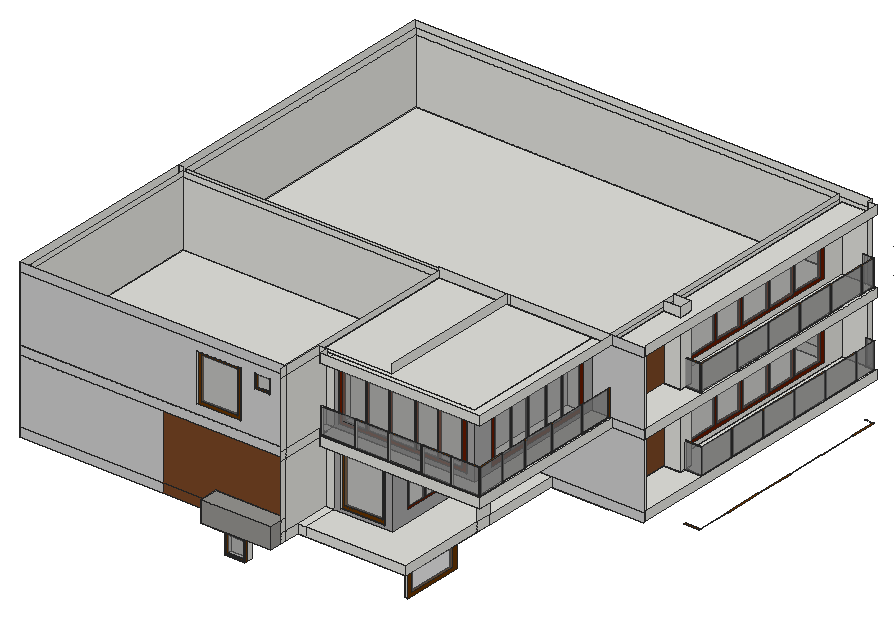
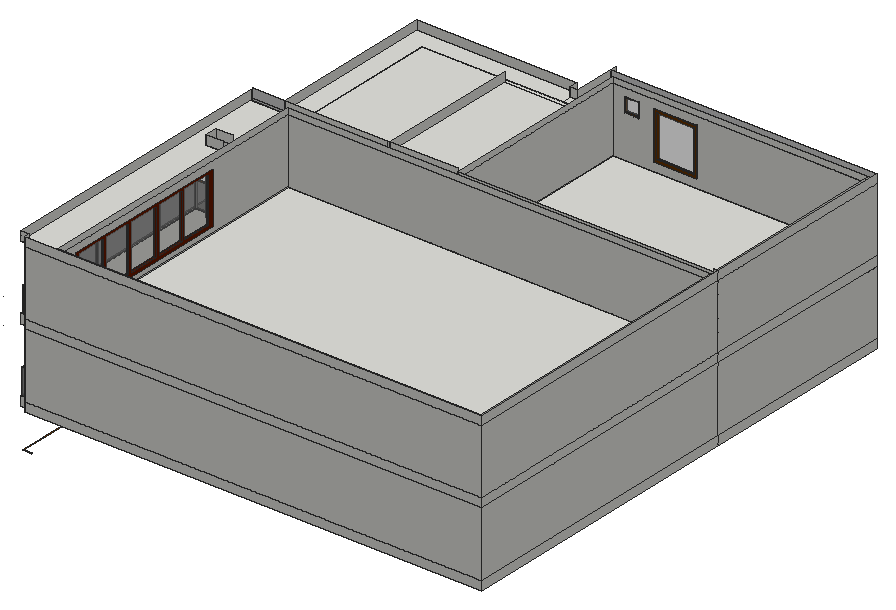
# SketchUp Ruby script. Lengths in inches.
U = 1.inch
M = Sketchup.active_model
def pt(a) = Geom::Point3d.new(a.map { |v| v * U })
def face(e, loops, mat)
  f = e.add_face(loops[0].map { |a| pt(a) })
  loops[1..].each { |l| e.add_face(l.map { |a| pt(a) }).erase! }
  f.material = f.back_material = mat if mat
  f
end
# faces: each face lists its corners as indices into pts; further lists are holes
def faces(e, pts, list, mat = nil) = list.each { |f| face(e, (f[0].is_a?(Array) ? f : [f]).map { |l| l.map { |i| pts[i] } }, mat) }
# xy, xz, yz: faces in a plane at the given z, y or x. An outline is a flat list of corners, or four numbers for a rectangle; further outlines are holes
def ring(l) = l.size == 4 ? [[l[0], l[1]], [l[2], l[1]], [l[2], l[3]], [l[0], l[3]]] : l.each_slice(2).to_a
def flat(e, list, mat, &to3) = list.each { |f| face(e, (f[0].is_a?(Array) ? f : [f]).map { |l| ring(l).map { |u, v| to3.(u, v) } }, mat) }
def xy(e, z, list, mat = nil) = flat(e, list, mat) { |x, y| [x, y, z] }
def xz(e, y, list, mat = nil) = flat(e, list, mat) { |x, z| [x, y, z] }
def yz(e, x, list, mat = nil) = flat(e, list, mat) { |y, z| [x, y, z] }
def lines(e, pts, list) = list.each { |a, b| e.add_line(pt(pts[a]), pt(pts[b])) }
# prism: a flat outline (further loops are holes) pulled along v
def prism(e, loops, v, mat = nil)
  f = face(e, loops, mat); d = Geom::Vector3d.new(v.map { |x| x * U })
  f.pushpull(f.normal.samedirection?(d) ? d.length : -d.length)
end
def box(e, o, s, mat = nil) = prism(e, [[o, [o[0] + s[0], o[1], o[2]], [o[0] + s[0], o[1] + s[1], o[2]], [o[0], o[1] + s[1], o[2]]]], [0, 0, s[2]], mat)
def at(x, y, z, deg = 0) = Geom::Transformation.translation(pt([x, y, z])) * Geom::Transformation.rotation(ORIGIN, Z_AXIS, deg.degrees)
def axes(o, x, y, z) = Geom::Transformation.new([*x, 0, *y, 0, *z, 0, *pt(o).to_a, 1])
def part(name) = M.definitions.add(name)
# library, detail: a bought-in or finely detailed component or shape, given as its bounding box
def library(name, o, s) = part(name).tap { |d| box(d.entities, o, s) }
def detail(e, o, s) = box(e.add_group.entities, o, s)
def put(e, d, t, mat = nil) = e.add_instance(d, t).tap { |i| i.material = mat if mat }
def group(e, t, mat = nil) = e.add_group.tap { |g| g.transformation = t; g.material = mat if mat }.entities
root = M.entities
M.materials.add("[Carrera Marble]").color = [207, 207, 207]
M.materials.add("[Color B08]").color = [102, 25, 0]
M.materials.add("[Color C08]").color = [102, 51, 0]
M.materials.add("[Granite Light Gray]").color = [149, 148, 144]
M.materials.add("[Stone Vein Gray]").color = [166, 165, 165]
M.materials.add("[Translucent Glass Gray]").color = [128, 128, 128]
M.materials["[Translucent Glass Gray]"].alpha = 0.5
M.materials.add("[Wood Veneer 01]").color = [120, 70, 37]
c1 = part("Group\#1")
xy(c1.entities,0,[[0,0,21.625,260.4375]],"[Color C08]")
xy(c1.entities,20.42,[[0,20.42,21.625,240.02]],"[Color C08]")
xy(c1.entities,312.95,[[0,20.42,21.625,240.02]],"[Color C08]")
xy(c1.entities,333.375,[[0,0,21.625,260.4375]],"[Color C08]")
xz(c1.entities,0,[[0,0,21.625,333.375]],"[Color C08]")
xz(c1.entities,20.42,[[0,20.42,21.625,312.95]],"[Color C08]")
xz(c1.entities,240.02,[[0,20.42,21.625,312.95]],"[Color C08]")
xz(c1.entities,260.4375,[[0,0,21.625,333.375]],"[Color C08]")
yz(c1.entities,0,[[[0,0,260.4375,333.375],[20.42,20.42,240.02,312.95]]],"[Color C08]")
yz(c1.entities,21.625,[[[0,0,260.4375,333.375],[20.42,20.42,240.02,312.95]]],"[Color C08]")
yz(c1.entities,21.625,[[20.42,20.42,240.02,312.95]],"[Translucent Glass Gray]")
c2 = part("Group\#3")
xy(c2.entities,0,[[0,0,23.0625,440.625]],"[Color B08]")
xy(c2.entities,14.28,[[0,14.28,23.0625,92.65],[0,98.4,23.0625,173.71],[0,179.46,23.0625,261.65],[0,267.4,23.0625,340.59],[0,346.34,23.0625,426.35]],"[Color B08]")
xy(c2.entities,204.03,[[0,14.28,23.0625,92.65],[0,98.4,23.0625,173.71],[0,179.46,23.0625,261.65],[0,267.4,23.0625,340.59],[0,346.34,23.0625,426.35]],"[Color B08]")
xy(c2.entities,218.3125,[[0,0,23.0625,440.625]],"[Color B08]")
xz(c2.entities,0,[[0,0,23.0625,218.3125]],"[Color B08]")
xz(c2.entities,14.28,[[0,14.28,23.0625,204.03]],"[Color B08]")
xz(c2.entities,92.65,[[0,14.28,23.0625,204.03]],"[Color B08]")
xz(c2.entities,98.4,[[0,14.28,23.0625,204.03]],"[Color B08]")
xz(c2.entities,173.71,[[0,14.28,23.0625,204.03]],"[Color B08]")
xz(c2.entities,179.46,[[0,14.28,23.0625,204.03]],"[Color B08]")
xz(c2.entities,261.65,[[0,14.28,23.0625,204.03]],"[Color B08]")
xz(c2.entities,267.4,[[0,14.28,23.0625,204.03]],"[Color B08]")
xz(c2.entities,340.59,[[0,14.28,23.0625,204.03]],"[Color B08]")
xz(c2.entities,346.34,[[0,14.28,23.0625,204.03]],"[Color B08]")
xz(c2.entities,426.35,[[0,14.28,23.0625,204.03]],"[Color B08]")
xz(c2.entities,440.625,[[0,0,23.0625,218.3125]],"[Color B08]")
yz(c2.entities,0,[[[0,0,440.625,218.3125],[179.46,14.28,261.65,204.03],[346.34,14.28,426.35,204.03],[14.28,14.28,92.65,204.03],[98.4,14.28,173.71,204.03],[267.4,14.28,340.59,204.03]]],"[Color B08]")
yz(c2.entities,23.0625,[[[0,0,440.625,218.3125],[179.46,14.28,261.65,204.03],[346.34,14.28,426.35,204.03],[14.28,14.28,92.65,204.03],[98.4,14.28,173.71,204.03],[267.4,14.28,340.59,204.03]]],"[Color B08]")
yz(c2.entities,23.0625,[[14.28,14.28,92.65,204.03],[98.4,14.28,173.71,204.03],[179.46,14.28,261.65,204.03],[267.4,14.28,340.59,204.03],[346.34,14.28,426.35,204.03]],"[Translucent Glass Gray]")
xy(root,566.178,[[607.75,336.9375,613.75,449.375]])
xy(root,603,[[828.5625,706.6875,856.375,711.1875],[856.375,706.6875,857.6875,711.1875],[856.375,711.1875,857.6875,772.085],[856.375,772.085,857.6875,773.74],[856.375,773.74,857.6875,844.71],
  [856.375,844.71,857.6875,846.365],[856.375,846.365,857.6875,917.335],[856.375,917.335,857.6875,918.99],[856.375,918.99,857.6875,989.96],[856.375,989.96,857.6875,991.615],
  [856.375,991.615,857.6875,1062.585],[856.375,1062.585,857.6875,1064.24],[856.375,1064.24,857.6875,1110],[841.515,1110,856.375,1110.8125],[856.375,1110,857.6875,1110.8125]],"[Color C08]")
xy(root,638.3125,[[406.64,171.6875,444.077,187]])
xy(root,659.99,[[607.75,336.9375,613.75,449.375]])
xy(root,661.371,[[791.375,750.158,797.375,1072.783]])
xy(root,667.778,[[517.666,301.1875,599.791,308.3125]])
xy(root,669,[[9,579,791.375,1111.6875]])
xy(root,675,[[9,579,791.375,1111.6875],[797.375,579,797.375,699.063,828.5625,699.063,828.5625,723.022,797.375,723.022,797.375,1111.6875,861.375,1111.6875,861.375,579]])
xy(root,675.75,[[362.246,171.6875,362.246,207.0625,491.3125,207.0625,491.3125,171.6875,444.077,171.6875,444.077,187,406.64,187,406.64,171.6875],[406.64,171.6875,444.077,187],[0,207.0625,0,573,9,573,9,213.0625,482.6875,213.0625,482.6875,308.3125,607.75,308.3125,607.75,573,613.75,573,613.75,301.1875,491.3125,301.1875,491.3125,207.0625],[491.3125,235.5625,506.0625,301.1875],[506.0625,235.5625,506.0625,301.1875,613.75,301.1875,613.75,573,691.028,573,691.028,235.5625]])
xy(root,686,[[9,213.0625,9,573,607.75,573,607.75,308.3125,482.6875,308.3125,482.6875,213.0625]])
xy(root,692,[[0,207.0625,0,573,9,573,9,213.0625,482.6875,213.0625,482.6875,308.3125,607.75,308.3125,607.75,573,613.75,573,613.75,301.1875,491.3125,301.1875,491.3125,207.0625],[9,213.0625,482.6875,213.0625,482.6875,308.3125,607.75,308.3125,607.75,573,9,573],[491.3125,235.5625,506.0625,301.1875],[506.0625,235.5625,691.028,235.5625,691.028,573,613.75,573,613.75,301.1875,506.0625,301.1875],[797.375,579,861.375,579,861.375,1111.6875,797.375,1111.6875,797.375,723.022,828.5625,723.022,828.5625,710.721,858.375,710.721,858.375,1109.6875,843.51,1109.6875,843.51,1110.875,859.875,1110.875,859.875,708.846,828.5625,708.846,828.5625,699.063,797.375,699.063],
  [828.5625,708.846,828.5625,710.721,858.375,710.721,858.375,779.522,859.875,779.522,859.875,708.846],[858.375,779.522,859.875,781.054],[858.375,781.054,859.875,851.647],[858.375,851.647,859.875,853.179],[858.375,853.179,859.875,923.772],
  [858.375,923.772,859.875,925.304],[858.375,925.304,859.875,995.897],[858.375,995.897,859.875,997.429],[858.375,997.429,859.875,1068.022],[858.375,1068.022,859.875,1069.554],
  [858.375,1069.554,858.375,1109.6875,843.51,1109.6875,843.51,1110.875,859.875,1110.875,859.875,1069.554]])
xy(root,697.447,[[517.451,301.1875,599.764,308.3125]])
xy(root,698.559,[[791.375,750.158,797.375,1072.783]])
xy(root,712.73,[[607.75,333.789,613.75,533.476]])
xy(root,714.625,[[362.246,171.6875,491.3125,207.0625]],"[Granite Light Gray]")
xy(root,740,[[828.5625,708.846,858.375,710.721],[858.375,708.846,859.875,710.721],[858.375,710.721,859.875,779.522],[858.375,779.522,859.875,781.054],[858.375,781.054,859.875,851.647],
  [858.375,851.647,859.875,853.179],[858.375,853.179,859.875,923.772],[858.375,923.772,859.875,925.304],[858.375,925.304,859.875,995.897],[858.375,995.897,859.875,997.429],
  [858.375,997.429,859.875,1068.022],[858.375,1068.022,859.875,1069.554],[858.375,1069.554,859.875,1069.554,859.875,1110.875,843.51,1110.875,843.51,1109.6875,858.375,1109.6875]],"[Color C08]")
xy(root,789.667,[[607.75,333.789,613.75,533.476]])
xy(root,797.434,[[791.375,750.158,797.375,1072.783]])
xy(root,800.572,[[517.451,301.1875,599.764,308.3125]])
xy(root,812,[[0,207.0625,0,573,9,573,9,213.0625,482.6875,213.0625,482.6875,308.3125,607.75,308.3125,607.75,573,613.75,573,613.75,301.1875,491.3125,301.1875,491.3125,207.0625],[[506.0625,267.5625,506.0625,301.1875,613.75,301.1875,613.75,573,801.71,573,801.71,267.5625],[691.028,400.901,719.841,429.151]],[491.3125,282.8125,506.0625,301.1875],[482.6875,308.3125,607.75,573],[691.028,400.901,719.841,429.151],
  [797.375,579,797.375,699.063,828.5625,699.063,828.5625,723.022,797.375,723.022,797.375,1111.6875,861.375,1111.6875,861.375,579]])
xy(root,822.125,[[9,213.0625,482.6875,573]])
xy(root,823,[[9,579,791.375,1111.6875]])
xy(root,829,[[0,207.0625,0,573,9,573,9,213.0625,482.6875,213.0625,482.6875,308.3125,607.75,308.3125,607.75,573,766.0625,573,766.0625,301.1875,491.3125,301.1875,491.3125,207.0625],[9,213.0625,482.6875,573],[506.0625,267.5625,801.71,267.5625,801.71,573,799.585,573,799.573,569.893,799.355,508.877,799.351,507.635,799.148,440.495,799.141,438.54,798.945,378.961,798.937,376.525,798.772,326.426,798.772,324.775,799.585,272.6875,799.585,270.6875,506.0625,270.6875],[506.0625,270.6875,508.257,272.6875],[508.257,270.6875,567.823,272.6875],
  [567.823,270.6875,569.893,272.6875],[569.893,270.6875,629.323,272.6875],[629.323,270.6875,631.393,272.6875],[631.393,270.6875,691.636,272.6875],[691.636,270.6875,693.706,272.6875],
  [693.706,270.6875,746.198,272.6875],[746.198,270.6875,748.268,272.6875],[748.268,270.6875,797.585,272.6875],[797.585,270.6875,797.779,272.6875],[797.779,270.6875,799.585,272.375],
  [797.779,272.375,799.585,272.6875],[506.0625,272.6875,691.636,272.6875,691.636,272.75,693.706,272.75,693.706,272.6875,797.585,272.6875,797.585,376.529,797.562,376.529,797.57,378.966,797.585,378.966,797.585,438.545,797.579,438.545,797.585,440.232,797.585,440.5,797.584,569.9,797.585,569.984,797.585,573,766.0625,573,766.0625,301.1875,506.0625,301.1875],[691.636,272.6875,693.706,272.75],[797.585,272.6875,797.585,324.775,798.772,324.775,799.585,272.6875],[491.3125,282.8125,506.0625,301.1875],
  [482.6875,308.3125,607.75,573],[797.585,324.775,798.772,326.426],[797.585,326.426,797.585,376.529,798.937,376.525,798.772,326.426],[798.937,376.525,797.585,376.529,797.585,378.966,798.945,378.961],[797.562,376.529,797.57,378.966,797.585,378.966,797.585,376.529],
  [798.945,378.961,797.585,378.966,797.585,438.545,799.141,438.54],[799.141,438.54,797.585,438.545,797.585,440.5,799.148,440.495],[797.579,438.545,797.585,438.545,797.585,440.232],[799.148,440.495,797.585,440.5,797.584,569.9,799.573,569.893,799.355,508.877,797.605,508.883,797.601,507.641,799.351,507.635],[799.351,507.635,797.601,507.641,797.605,508.883,799.355,508.877],
  [799.573,569.893,797.584,569.9,797.585,569.984,797.595,573,799.585,573],[797.585,569.984,797.585,573,797.595,573],[797.595,573,797.595,573.007,799.585,573],[9,579,791.375,1111.6875],[797.375,579,861.375,579,861.375,1111.6875,797.375,1111.6875,797.375,723.022,828.5625,723.022,828.5625,712.375,856.375,712.375,856.375,1109.385,838.579,1109.385,838.579,1110.448,858.125,1110.448,858.125,709.875,828.5625,709.875,828.5625,699.063,797.375,699.063],
  [828.5625,709.875,856.375,712.375],[856.375,709.875,858.125,712.375],[856.375,712.375,858.125,794.565],[856.375,794.565,858.125,796],[856.375,796,858.125,866.565],
  [856.375,866.565,858.125,868],[856.375,868,858.125,938.565],[856.375,938.565,858.125,940],[856.375,940,858.125,1010.565],[856.375,1010.565,858.125,1012],
  [856.375,1012,858.125,1082.565],[856.375,1082.565,858.125,1084],[856.375,1084,858.125,1109.385],[838.579,1109.385,856.375,1110.448],[856.375,1109.385,858.125,1110.448]])
xy(root,836.402,[[514.904,301.1875,750.717,325.5625]])
xy(root,836.699,[[736.6875,339.975,766.0625,551.413]])
xy(root,837.871,[[791.375,750.158,797.375,1072.783]])
xy(root,844.835,[[327.221,207.0625,407.721,213.0625]])
xy(root,877,[[691.636,272.6875,693.706,272.75],[797.562,376.529,797.585,376.529,797.585,378.966,797.57,378.966],[797.579,438.545,797.585,438.545,797.585,440.232],[797.585,569.984,797.595,573,797.585,573],[797.595,573,799.585,573,797.595,573.007]])
xy(root,877,[[506.0625,270.6875,508.257,272.6875],[508.257,270.6875,567.823,272.6875],[567.823,270.6875,569.893,272.6875],[569.893,270.6875,629.323,272.6875],[629.323,270.6875,631.393,272.6875],
  [631.393,270.6875,691.636,272.6875],[691.636,270.6875,693.706,272.6875],[693.706,270.6875,746.198,272.6875],[746.198,270.6875,748.268,272.6875],[748.268,270.6875,797.585,272.6875],
  [797.585,270.6875,799.585,272.6875],[797.585,272.6875,799.585,272.6875,798.772,324.775,797.585,324.775],[797.585,324.775,798.772,326.426],[797.585,326.426,798.772,326.426,798.937,376.525,797.585,376.529],[798.937,376.525,798.945,378.961,797.585,378.966,797.585,376.529],
  [798.945,378.961,799.141,438.54,797.585,438.545,797.585,378.966],[799.141,438.54,799.148,440.495,797.585,440.5,797.585,438.545],[799.148,440.495,799.351,507.635,797.601,507.641,797.605,508.883,799.355,508.877,799.573,569.893,797.584,569.9,797.585,440.5],[799.351,507.635,799.355,508.877,797.605,508.883,797.601,507.641],[799.573,569.893,799.585,573,797.595,573,797.585,569.984,797.584,569.9],
  [828.5625,709.875,856.375,712.375],[856.375,709.875,858.125,712.375],[856.375,712.375,858.125,794.565],[856.375,794.565,858.125,796],[856.375,796,858.125,866.565],
  [856.375,866.565,858.125,868],[856.375,868,858.125,938.565],[856.375,938.565,858.125,940],[856.375,940,858.125,1010.565],[856.375,1010.565,858.125,1012],
  [856.375,1012,858.125,1082.565],[856.375,1082.565,858.125,1084],[856.375,1084,858.125,1109.385],[838.579,1109.385,856.375,1110.448],[856.375,1109.385,858.125,1110.448]],"[Color C08]")
xy(root,907.498,[[434.387,207.0625,461.574,213.0625]])
xy(root,933.199,[[736.6875,339.975,766.0625,551.413]])
xy(root,933.96,[[327.221,207.0625,407.721,213.0625]])
xy(root,934.686,[[434.387,207.0625,461.574,213.0625]])
xy(root,936.746,[[791.375,750.158,797.375,1072.783]])
xy(root,943.152,[[514.904,301.1875,750.717,325.5625]])
xy(root,949,[[0,207.0625,0,573,9,573,9,213.0625,482.6875,213.0625,482.6875,308.3125,607.75,308.3125,607.75,573,766.0625,573,766.0625,301.1875,491.3125,301.1875,491.3125,207.0625],[506.0625,267.5625,506.0625,301.1875,766.0625,301.1875,766.0625,573,801.71,573,801.71,267.5625],[491.3125,282.8125,506.0625,301.1875],[482.6875,308.3125,607.75,573],[797.375,579,797.375,699.063,828.5625,699.063,828.5625,723.022,797.375,723.022,797.375,1111.6875,861.375,1111.6875,861.375,579]])
xz(root,171.6875,[[362.246,675.75,491.3125,714.625]],"[Granite Light Gray]")
xz(root,187,[[406.64,638.3125,444.077,675.75]])
xz(root,207.0625,[[362.246,675.75,491.3125,692],[362.246,692,491.3125,714.625]])
xz(root,207.0625,[[0,675.75,263.742,692],[0,692,263.742,812],[0,812,491.3125,829],[[0,829,491.3125,949],[327.221,844.835,407.721,933.96],[434.387,907.498,461.574,934.686]],[0,949,491.3125,966]],"[Carrera Marble]")
xz(root,207.0625,[[263.742,675.75,362.246,692],[263.742,692,362.246,692,362.246,714.625,491.3125,714.625,491.3125,812,263.742,812]],"[Wood Veneer 01]")
xz(root,213.0625,[[9,675.75,482.6875,686],[9,686,482.6875,692],[9,692,482.6875,812],[9,812,482.6875,822.125],[9,822.125,482.6875,829],
  [[9,829,482.6875,949],[327.221,844.835,407.721,933.96],[434.387,907.498,461.574,934.686]],[9,949,482.6875,960]])
xz(root,235.5625,[[491.3125,675.75,506.0625,692],[506.0625,675.75,691.028,692]])
xz(root,267.5625,[[506.0625,812,801.71,829],[506.0625,949,801.71,966]])
xz(root,270.6875,[[506.0625,829,508.257,877],[567.823,829,569.893,877],[629.323,829,631.393,877],[691.636,829,693.706,877],[746.198,829,748.268,877],
  [797.585,829,799.585,877]],"[Color C08]")
xz(root,270.6875,[[508.257,829,567.823,877],[569.893,829,629.323,877],[631.393,829,691.636,877],[693.706,829,746.198,877],[748.268,829,797.585,877]],"[Translucent Glass Gray]")
xz(root,272.6875,[[797.585,829,799.585,877]])
xz(root,272.6875,[[567.823,829,569.893,877],[629.323,829,631.393,877],[746.198,829,748.268,877]],"[Color C08]")
xz(root,272.6875,[[508.257,829,567.823,877],[569.893,829,629.323,877],[631.393,829,746.198,877],[748.268,829,797.585,877]],"[Translucent Glass Gray]")
xz(root,272.75,[[691.636,829,693.706,877]],"[Color C08]")
xz(root,282.8125,[[491.3125,812,506.0625,829],[491.3125,949,506.0625,966]])
xz(root,301.1875,[[491.3125,692,506.0625,812],[491.3125,829,506.0625,949]])
xz(root,301.1875,[[[506.0625,692,613.75,812],[517.451,697.447,599.764,800.572]],[[506.0625,829,766.0625,949],[514.904,836.402,750.717,943.152]]],"[Stone Vein Gray]")
xz(root,308.3125,[[482.6875,675.75,607.75,686],[482.6875,686,607.75,692],[[482.6875,692,607.75,812],[517.451,697.447,599.764,800.572]],[482.6875,812,607.75,829]])
xz(root,324.775,[[797.585,829,798.772,877]])
xz(root,325.5625,[[514.904,836.402,750.717,943.152]])
xz(root,326.426,[[797.585,829,798.772,877]])
xz(root,333.789,[[607.75,712.73,613.75,789.667]])
xz(root,336.9375,[[607.75,566.178,613.75,659.99]])
xz(root,339.975,[[736.6875,836.699,766.0625,933.199]])
xz(root,449.375,[[607.75,566.178,613.75,659.99]])
xz(root,533.476,[[607.75,712.73,613.75,789.667]])
xz(root,551.413,[[736.6875,836.699,766.0625,933.199]])
xz(root,573,[[0,675,9,675.75],[9,675,607.75,686],[607.75,675,613.75,675.75],[0,675.75,9,692],[607.75,675.75,691.028,692],
  [9,686,607.75,692],[0,692,9,812],[9,692,607.75,812],[607.75,692,613.75,812],[0,812,9,829],
  [9,812,482.6875,822.125],[482.6875,812,607.75,829],[607.75,812,613.75,829],[613.75,812,801.71,829],[9,822.125,482.6875,829],
  [0,829,9,949],[9,829,482.6875,949],[482.6875,829,607.75,949],[607.75,829,766.0625,949],[797.585,829,799.585,877],
  [0,949,9,966],[9,949,482.6875,960],[482.6875,949,607.75,966],[607.75,949,613.75,966],[613.75,949,801.71,966]])
xz(root,573,[[613.75,675,861.375,675,861.375,692,691.028,692,691.028,675.75,613.75,675.75],[613.75,692,861.375,812],[801.71,812,861.375,829],[766.0625,829,797.585,829,797.585,877,799.585,877,799.585,829,861.375,829,861.375,949,766.0625,949],[801.71,949,861.375,966]],"[Carrera Marble]")
xz(root,579,[[9,669,791.375,675],[9,675,791.375,692],[797.375,675,861.375,692],[9,692,791.375,812],[797.375,692,861.375,812],
  [9,812,791.375,823],[9,823,791.375,829],[9,829,791.375,949],[797.375,829,861.375,949],[9,949,791.375,960]])
xz(root,699.063,[[797.375,675,828.5625,692],[797.375,692,828.5625,812],[797.375,812,828.5625,829],[797.375,829,828.5625,949],[797.375,949,828.5625,966]])
xz(root,708.846,[[828.5625,692,859.875,740]],"[Translucent Glass Gray]")
xz(root,709.875,[[856.375,829,858.125,877]],"[Color C08]")
xz(root,709.875,[[828.5625,829,856.375,877]],"[Translucent Glass Gray]")
xz(root,710.721,[[828.5625,692,858.375,740]],"[Translucent Glass Gray]")
xz(root,712.375,[[856.375,829,858.125,877]])
xz(root,712.375,[[828.5625,829,856.375,877]],"[Translucent Glass Gray]")
xz(root,723.022,[[797.375,675,828.5625,692],[797.375,692,828.5625,812],[797.375,812,828.5625,829],[797.375,829,828.5625,949],[797.375,949,828.5625,966]])
xz(root,750.158,[[791.375,698.559,797.375,797.434],[791.375,837.871,797.375,936.746]])
xz(root,779.522,[[858.375,692,859.875,740]])
xz(root,781.054,[[858.375,692,859.875,740]])
xz(root,794.565,[[856.375,829,858.125,877]])
xz(root,796,[[856.375,829,858.125,877]])
xz(root,851.647,[[858.375,692,859.875,740]])
xz(root,853.179,[[858.375,692,859.875,740]])
xz(root,866.565,[[856.375,829,858.125,877]])
xz(root,868,[[856.375,829,858.125,877]])
xz(root,923.772,[[858.375,692,859.875,740]])
xz(root,925.304,[[858.375,692,859.875,740]])
xz(root,938.565,[[856.375,829,858.125,877]])
xz(root,940,[[856.375,829,858.125,877]])
xz(root,995.897,[[858.375,692,859.875,740]])
xz(root,997.429,[[858.375,692,859.875,740]])
xz(root,1010.565,[[856.375,829,858.125,877]])
xz(root,1012,[[856.375,829,858.125,877]])
xz(root,1068.022,[[858.375,692,859.875,740]])
xz(root,1069.554,[[858.375,692,859.875,740]])
xz(root,1072.783,[[791.375,698.559,797.375,797.434],[791.375,837.871,797.375,936.746]])
xz(root,1082.565,[[856.375,829,858.125,877]])
xz(root,1084,[[856.375,829,858.125,877]])
xz(root,1109.385,[[856.375,829,858.125,877]])
xz(root,1109.385,[[838.579,829,856.375,877]],"[Translucent Glass Gray]")
xz(root,1109.6875,[[843.51,692,858.375,740]],"[Translucent Glass Gray]")
xz(root,1110.448,[[856.375,829,858.125,877]],"[Color C08]")
xz(root,1110.448,[[838.579,829,856.375,877]],"[Translucent Glass Gray]")
xz(root,1110.875,[[843.51,692,859.875,740]],"[Translucent Glass Gray]")
xz(root,1111.6875,[[9,669,791.375,675],[9,675,791.375,692],[797.375,675,845.0625,692],[845.0625,675,861.375,692],[9,692,791.375,812],
  [797.375,692,845.0625,812],[9,812,791.375,823],[845.0625,812,861.375,829],[9,823,791.375,829],[9,829,791.375,949],
  [797.375,829,845.0625,949],[9,949,791.375,960],[845.0625,949,861.375,966]])
xz(root,1120.6875,[[0,675,845.0625,692],[0,692,845.0625,812],[0,812,845.0625,829],[0,829,845.0625,949],[0,949,845.0625,966]])
yz(root,0,[[573,675,1120.6875,692],[207.0625,675.75,573,692],[207.0625,692,573,812],[573,692,1120.6875,812],[207.0625,812,573,829],
  [573,812,1120.6875,829],[207.0625,829,573,949],[573,829,1120.6875,949],[207.0625,949,573,966],[573,949,1120.6875,966]])
yz(root,9,[[579,669,1111.6875,675],[579,675,1111.6875,692],[213.0625,675.75,222,686],[222,675.75,573,686],[213.0625,686,222,692],
  [222,686,573,692],[213.0625,692,222,812],[222,692,573,812],[579,692,1111.6875,812],[213.0625,812,222,822.125],
  [222,812,573,822.125],[579,812,1111.6875,823],[213.0625,822.125,222,829],[222,822.125,573,829],[579,823,1111.6875,829],
  [213.0625,829,222,949],[222,829,573,949],[579,829,1111.6875,949],[213.0625,949,222,960],[222,949,573,960],
  [579,949,1111.6875,960]])
yz(root,327.221,[[207.0625,844.835,213.0625,933.96]])
yz(root,362.246,[[171.6875,675.75,207.0625,714.625]],"[Granite Light Gray]")
yz(root,406.64,[[171.6875,638.3125,187,675.75]])
yz(root,407.721,[[207.0625,844.835,213.0625,933.96]])
yz(root,434.387,[[207.0625,907.498,213.0625,934.686]])
yz(root,444.077,[[171.6875,638.3125,187,675.75]])
yz(root,461.574,[[207.0625,907.498,213.0625,934.686]])
yz(root,482.6875,[[213.0625,675.75,308.3125,686],[213.0625,686,260.6875,692],[260.6875,686,280.785,692],[280.785,686,308.3125,692],[213.0625,692,308.3125,812],
  [213.0625,812,308.3125,822.125],[308.3125,812,573,822.125],[213.0625,822.125,288.5625,829],[288.5625,822.125,308.3125,829],[308.3125,822.125,573,829],
  [213.0625,829,573,949],[213.0625,949,573,960]])
yz(root,491.3125,[[195.6875,675.75,207.0625,692],[207.0625,675.75,235.5625,692],[195.6875,692,207.0625,714.625],[207.0625,692,301.1875,812],[195.6875,714.625,207.0625,812],
  [195.6875,812,207.0625,829],[207.0625,812,282.8125,829],[195.6875,829,207.0625,949],[207.0625,829,301.1875,949],[195.6875,949,207.0625,966],
  [207.0625,949,282.8125,966]])
yz(root,491.3125,[[171.6875,675.75,195.6875,714.625]],"[Granite Light Gray]")
yz(root,506.0625,[[267.5625,812,282.8125,829],[267.5625,949,282.8125,966]])
yz(root,506.0625,[[270.6875,829,272.6875,877]],"[Color C08]")
yz(root,508.257,[[270.6875,829,272.6875,877]])
yz(root,514.904,[[301.1875,836.402,325.5625,943.152]])
yz(root,517.451,[[301.1875,697.447,308.3125,800.572]])
yz(root,567.823,[[270.6875,829,272.6875,877]])
yz(root,569.893,[[270.6875,829,272.6875,877]])
yz(root,599.764,[[301.1875,697.447,308.3125,800.572]])
yz(root,607.75,[[308.3125,675.75,573,686],[308.3125,686,573,692],[[308.3125,692,573,812],[333.789,712.73,533.476,789.667]],[308.3125,812,573,829],[308.3125,949,573,966]])
yz(root,613.75,[[[301.1875,692,538.722,812],[333.789,712.73,533.476,789.667]]],"[Stone Vein Gray]")
yz(root,613.75,[[538.722,692,573,812]],"[Wood Veneer 01]")
yz(root,629.323,[[270.6875,829,272.6875,877]])
yz(root,631.393,[[270.6875,829,272.6875,877]])
yz(root,691.028,[[235.5625,675.75,400.901,692],[400.901,675.75,429.151,692],[429.151,675.75,573,692],[400.901,692,429.151,812]])
yz(root,691.636,[[270.6875,829,272.75,877]])
yz(root,693.706,[[270.6875,829,272.75,877]])
yz(root,736.6875,[[339.975,836.699,551.413,933.199]])
yz(root,746.198,[[270.6875,829,272.6875,877]])
yz(root,748.268,[[270.6875,829,272.6875,877]])
yz(root,750.717,[[301.1875,836.402,325.5625,943.152]])
yz(root,766.0625,[[[301.1875,829,573,949],[339.975,836.699,551.413,933.199]]],"[Stone Vein Gray]")
yz(root,791.375,[[579,669,721.796,675],[721.796,669,734.483,675],[734.483,669,1111.6875,675],[[579,675,1111.6875,823],[750.158,698.559,1072.783,797.434]],[579,823,1111.6875,829],
  [[579,829,1111.6875,949],[750.158,837.871,1072.783,936.746]],[579,949,1111.6875,960]])
yz(root,797.375,[[579,675,699.063,692],[723.022,675,1111.6875,692],[[723.022,692,1111.6875,812],[750.158,698.559,1072.783,797.434]],[[723.022,829,1111.6875,949],[750.158,837.871,1072.783,936.746]]])
yz(root,797.375,[[579,692,699.063,812],[579,829,699.063,949]],"[Wood Veneer 01]")
yz(root,797.585,[[270.6875,829,272.6875,877]])
yz(root,797.585,[[324.775,829,326.426,877]],"[Color C08]")
yz(root,797.585,[[272.6875,829,324.775,877],[326.426,829,440.5,877]],"[Translucent Glass Gray]")
yz(root,798.772,[[324.775,829,326.426,877]],"[Color C08]")
yz(root,799.585,[[270.6875,829,272.6875,877]],"[Color C08]")
yz(root,801.71,[[267.5625,812,573,829],[267.5625,949,573,966]])
yz(root,828.5625,[[699.063,675,723.022,692],[699.063,692,708.846,692,708.846,740,710.721,740,710.721,692,723.022,692,723.022,812,699.063,812],[708.846,692,710.721,740],[699.063,812,723.022,829],[699.063,829,709.875,829,709.875,877,712.375,877,712.375,829,723.022,829,723.022,949,699.063,949],
  [709.875,829,712.375,877],[699.063,949,723.022,966]])
yz(root,838.579,[[1109.385,829,1110.448,877]])
yz(root,843.51,[[1109.6875,692,1110.875,740]])
yz(root,845.0625,[[1111.6875,675,1120.6875,692],[1111.6875,692,1120.6875,812],[1111.6875,812,1120.6875,829],[1111.6875,829,1120.6875,949],[1111.6875,949,1120.6875,966]])
yz(root,856.375,[[709.875,829,712.375,877],[1109.385,829,1110.448,877]])
yz(root,856.375,[[794.565,829,796,877],[866.565,829,868,877],[938.565,829,940,877],[1010.565,829,1012,877],[1082.565,829,1084,877]],"[Color C08]")
yz(root,856.375,[[712.375,829,794.565,877],[796,829,866.565,877],[868,829,938.565,877],[940,829,1010.565,877],[1012,829,1082.565,877],
  [1084,829,1109.385,877]],"[Translucent Glass Gray]")
yz(root,858.125,[[709.875,829,712.375,877],[794.565,829,796,877],[866.565,829,868,877],[938.565,829,940,877],[1010.565,829,1012,877],
  [1082.565,829,1084,877],[1109.385,829,1110.448,877]],"[Color C08]")
yz(root,858.125,[[712.375,829,794.565,877],[796,829,866.565,877],[868,829,938.565,877],[940,829,1010.565,877],[1012,829,1082.565,877],
  [1084,829,1109.385,877]],"[Translucent Glass Gray]")
yz(root,858.375,[[779.522,692,781.054,740],[851.647,692,853.179,740],[923.772,692,925.304,740],[995.897,692,997.429,740],[1068.022,692,1069.554,740]],"[Color C08]")
yz(root,858.375,[[710.721,692,779.522,740],[781.054,692,851.647,740],[853.179,692,923.772,740],[925.304,692,995.897,740],[997.429,692,1068.022,740],
  [1069.554,692,1109.6875,740]],"[Translucent Glass Gray]")
yz(root,859.875,[[708.846,692,710.721,740],[779.522,692,781.054,740],[851.647,692,853.179,740],[923.772,692,925.304,740],[995.897,692,997.429,740],
  [1068.022,692,1069.554,740]],"[Color C08]")
yz(root,859.875,[[710.721,692,779.522,740],[781.054,692,851.647,740],[853.179,692,923.772,740],[925.304,692,995.897,740],[997.429,692,1068.022,740],
  [1069.554,692,1110.875,740]],"[Translucent Glass Gray]")
yz(root,861.375,[[579,675,1111.6875,692],[579,812,1111.6875,829],[579,949,1111.6875,966]])
p = [[799.585,272.6875,829],[798.772,324.775,829],[798.772,324.775,877],[799.585,272.6875,877],[798.772,326.426,829],[798.937,376.525,829],
  [798.937,376.525,877],[798.772,326.426,877],[797.57,378.966,829],[797.562,376.529,829],[797.562,376.529,877],[797.57,378.966,877],
  [797.585,376.529,877],[797.585,376.529,829],[798.945,378.961,829],[798.945,378.961,877],[797.585,378.966,829],[797.585,378.966,877],
  [799.141,438.54,829],[799.141,438.54,877],[797.585,440.5,829],[797.585,440.232,829],[797.579,438.545,829],[797.579,438.545,877],
  [797.585,440.232,877],[797.585,440.5,877],[797.585,438.545,877],[797.585,438.545,829],[799.148,440.495,829],[799.148,440.495,877],
  [797.584,569.9,877],[797.584,569.9,829],[799.351,507.635,829],[799.351,507.635,877],[797.605,508.883,829],[797.601,507.641,829],
  [797.601,507.641,877],[797.605,508.883,877],[799.355,508.877,829],[799.355,508.877,877],[799.573,569.893,829],[799.573,569.893,877],
  [797.595,573,877],[797.595,573.007,877],[797.595,573.007,829],[797.595,573,829],[797.585,569.984,829],[797.585,569.984,877],
  [797.585,573,877],[797.585,573,829],[799.585,573,877],[799.585,573,829],[797.779,272.375,877],[797.779,272.375,829],
  [858.125,1154.565,877],[858.125,1156,877],[858.125,1154.565,829],[858.125,1156,829]]
faces(root,p,[[0,1,2,3],[4,5,6,7],[14,18,19,15],[25,30,31,20],[28,32,33,29],[38,40,41,39]],"[Translucent Glass Gray]")
faces(root,p,[[8,9,10,11],[5,14,15,6],[20,21,22,23,24,25],[18,28,29,19],[32,38,39,33],[46,31,30,47,48,49],[50,41,40,51]],"[Color C08]")
faces(root,p,[[5,6,12,10,9,13],[15,14,16,8,11,17],[18,19,26,23,22,27],[29,28,20,25],[34,35,36,37],[32,33,36,35],[39,38,34,37],[42,43,44,45,46,31,30,47],
  [40,41,30,31],[50,51,44,43]])
lines(root,p,[[52,53],[54,55],[56,57]])
put(root,c1,axes([607.64,336.9375,566.18],[0.28,0,0],[0,0.43173,0],[0,0,0.28]))
put(root,c1,axes([406.64,173.97,638.3125],[0,0.11448,0],[0.14375,0,0],[0,0,0.1123]))
put(root,c1,axes([517.45,307.24,697.45],[0,-0.1652,0],[0.31605,0,0],[0,0,0.30934]))
put(root,c2,axes([792.53,750.55,698.56],[0.21,0,0],[0,0.7313,0],[0,0,0.45291]))
put(root,c2,axes([610.84,333.79,710.57],[0.09257,0,0],[0,0.45705,0],[0,0,0.36649]))
put(root,c2,axes([514.9,303.92,836.4],[0,-0.11844,0],[0.53518,0,0],[0,0,0.48898]))
put(root,c2,axes([763.93,339.98,836.7],[0.09257,0,0],[0,0.47986,0],[0,0,0.44203]))
put(root,c2,axes([792.53,750.55,837.87],[0.21,0,0],[0,0.7313,0],[0,0,0.45291]))
put(root,c1,axes([327.22,213.12,844.83],[0,-0.1652,0],[0.3091,0,0],[0,0,0.26597]))
put(root,c1,axes([434.39,209.34,907.5],[0,0.11448,0],[0.10439,0,0],[0,0,0.08155]))
